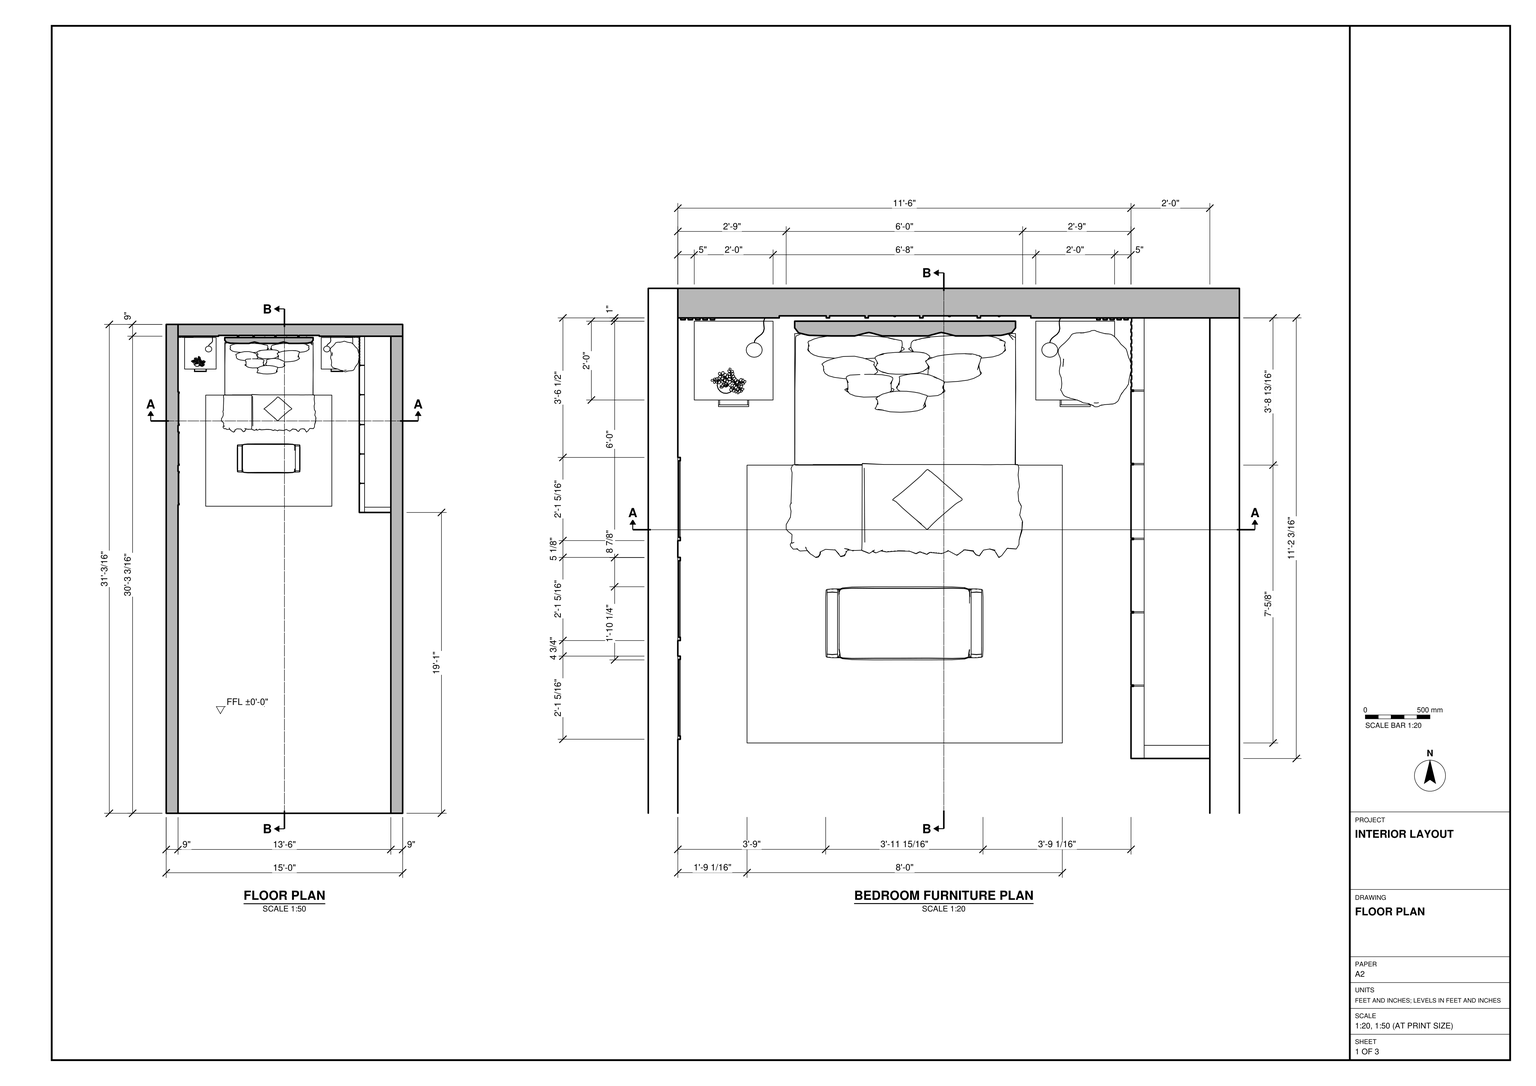
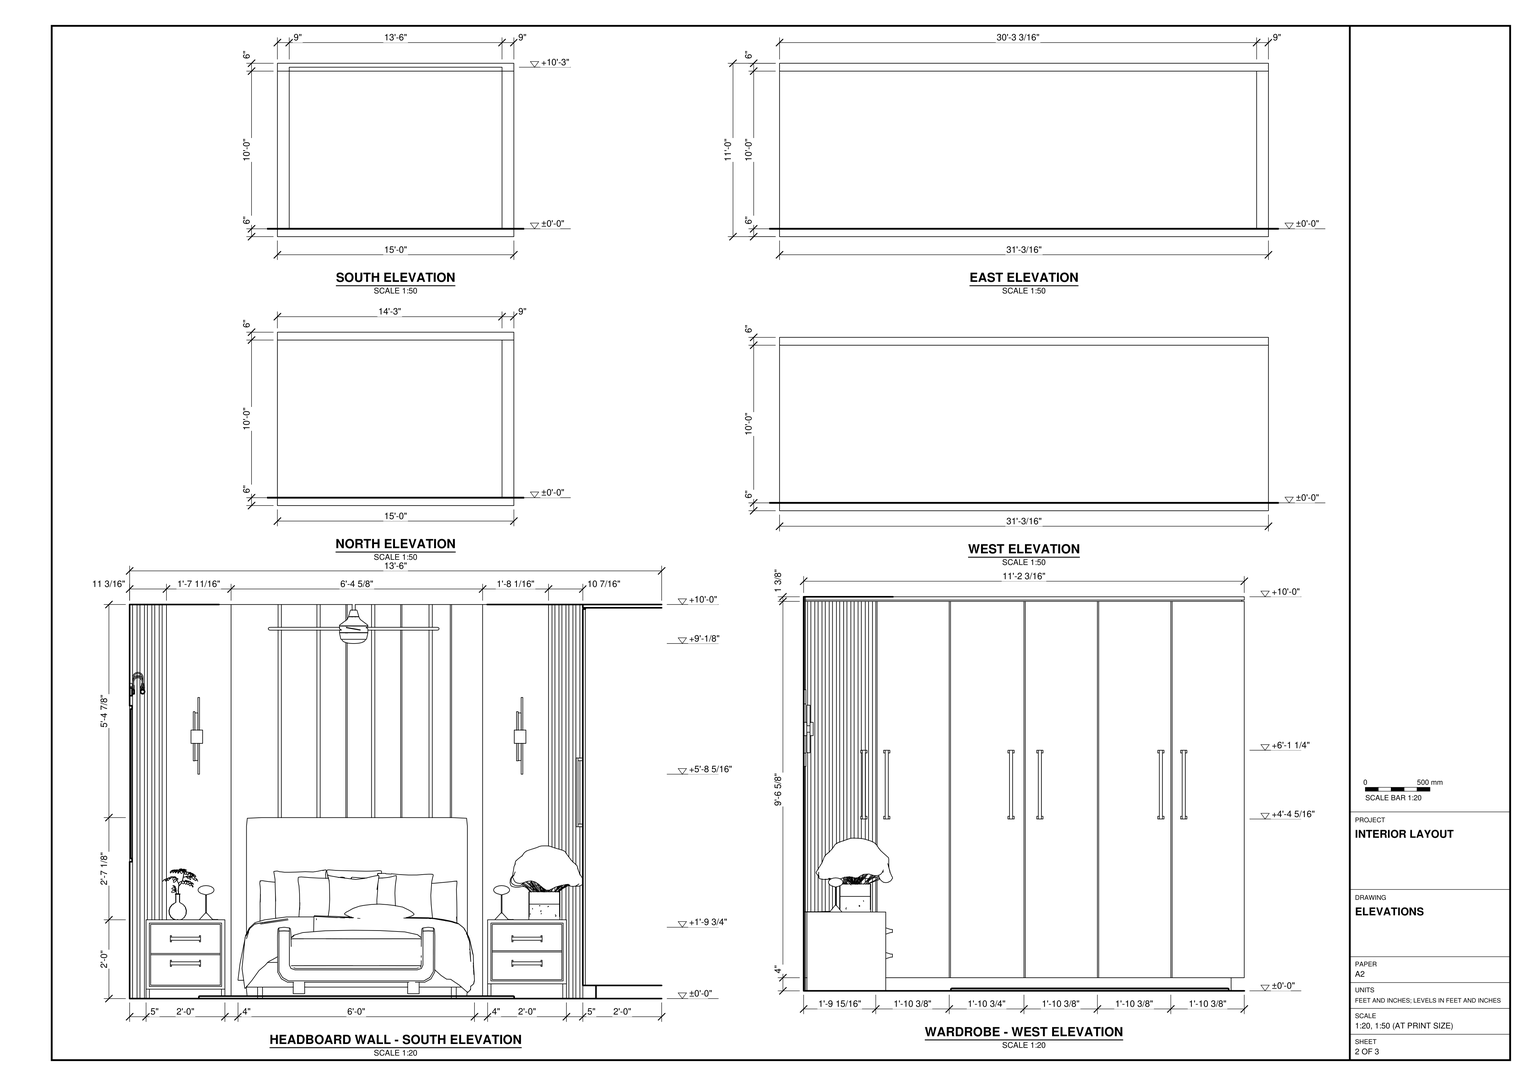
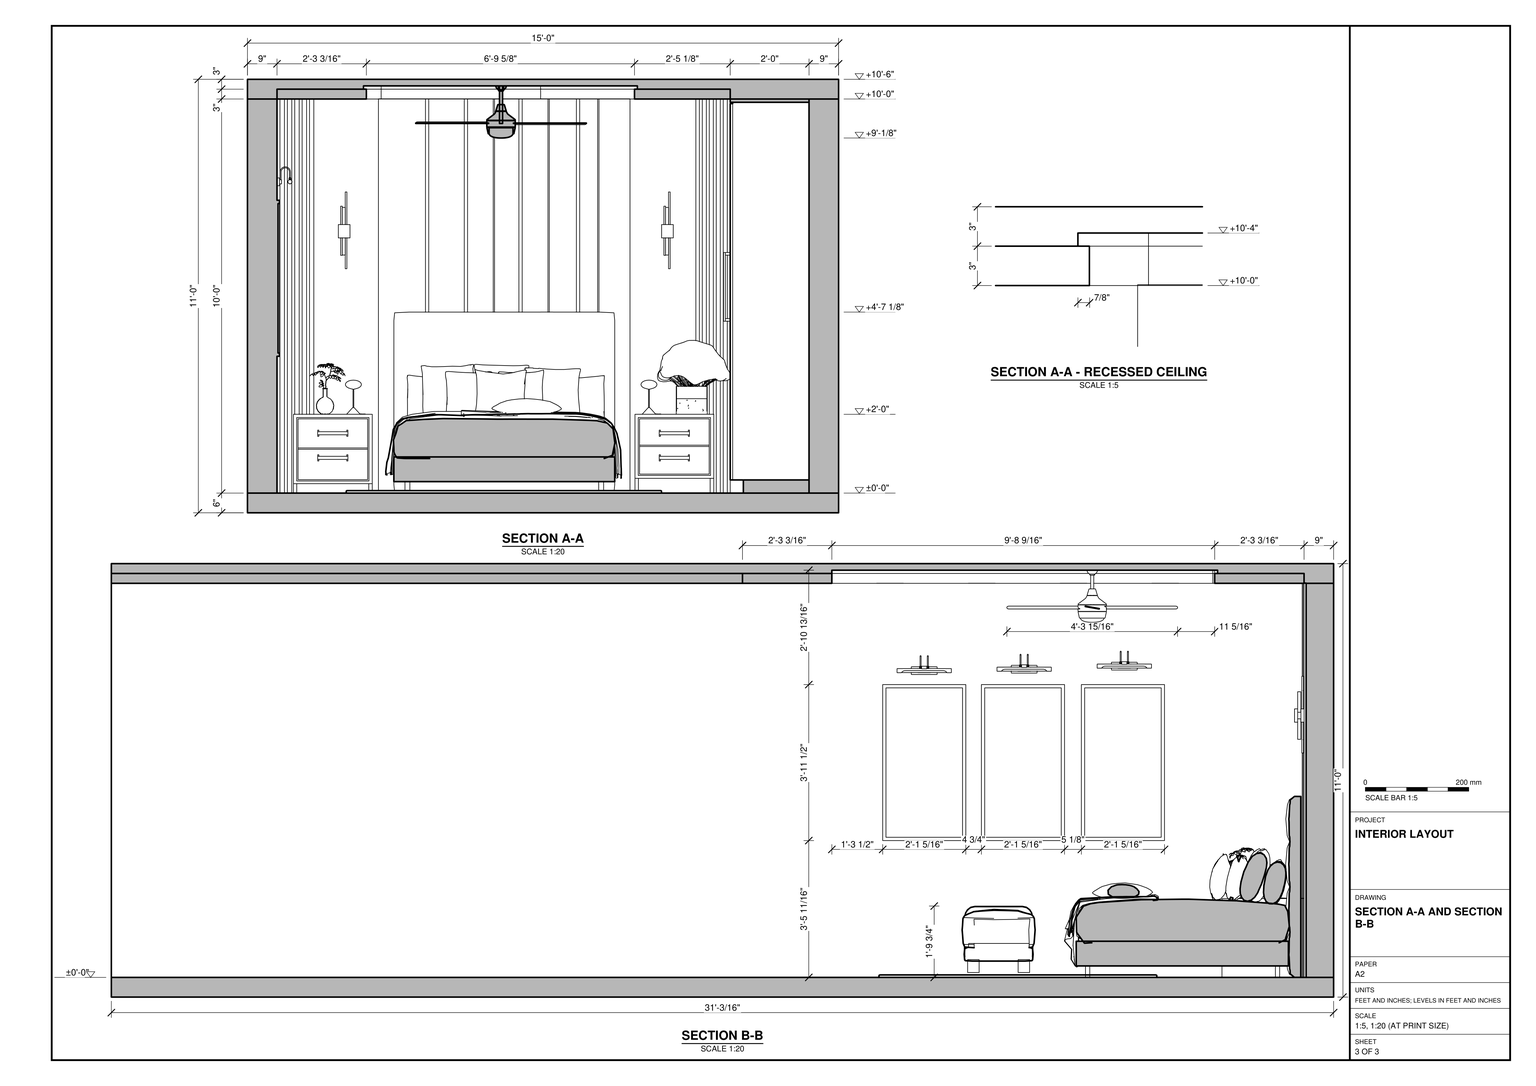
Work in feet and inches. Use task_files/diagram_01.pdf to build the bedroom in SketchUp. Set the finished floor at ±0'-0" and make the shell 15'-0" wide, 31'-3/16" long and 11'-0" high overall. Build the floor slab, the two long side walls, the headboard wall and the upper slab. Use the wall and slab thicknesses shown in section. Leave the end opposite the headboard open as drawn.

Use the enlarged furniture plan to place the bed between the bedside drawer units, with the fitted wardrobe running along the adjacent side wall. Centre the bench across the foot of the bed and place the rug beneath the bench and the foot of the bed. Keep the remaining length of the room clear. Follow the elevations for the headboard wall panelling, the wardrobe fronts, handles and recessed base. Use the sections to locate the stepped ceiling recess, ceiling fan, wall lights and framed panels.

Keep shell elements and individual furniture or joinery pieces in separate groups or components, and use components for repeated parts. Decor and loose items, including the rug, lamps and bedside objects, may be any suitable library components. Save one SketchUp model as output_files/bedroom_with_a_fitted_wardrobe_and_recessed_ceiling.skp.

# SketchUp Ruby script. Lengths in inches.
U = 1.inch
M = Sketchup.active_model
def pt(a) = Geom::Point3d.new(a.map { |v| v * U })
def face(e, loops, mat)
  f = e.add_face(loops[0].map { |a| pt(a) })
  loops[1..].each { |l| e.add_face(l.map { |a| pt(a) }).erase! }
  f.material = f.back_material = mat if mat
  f
end
# faces: each face lists its corners as indices into pts; further lists are holes
def faces(e, pts, list, mat = nil) = list.each { |f| face(e, (f[0].is_a?(Array) ? f : [f]).map { |l| l.map { |i| pts[i] } }, mat) }
# xy, xz, yz: faces in a plane at the given z, y or x. An outline is a flat list of corners, or four numbers for a rectangle; further outlines are holes
def ring(l) = l.size == 4 ? [[l[0], l[1]], [l[2], l[1]], [l[2], l[3]], [l[0], l[3]]] : l.each_slice(2).to_a
def flat(e, list, mat, &to3) = list.each { |f| face(e, (f[0].is_a?(Array) ? f : [f]).map { |l| ring(l).map { |u, v| to3.(u, v) } }, mat) }
def xy(e, z, list, mat = nil) = flat(e, list, mat) { |x, y| [x, y, z] }
def xz(e, y, list, mat = nil) = flat(e, list, mat) { |x, z| [x, y, z] }
def yz(e, x, list, mat = nil) = flat(e, list, mat) { |y, z| [x, y, z] }
def lines(e, pts, list) = list.each { |a, b| e.add_line(pt(pts[a]), pt(pts[b])) }
# prism: a flat outline (further loops are holes) pulled along v
def prism(e, loops, v, mat = nil)
  f = face(e, loops, mat); d = Geom::Vector3d.new(v.map { |x| x * U })
  f.pushpull(f.normal.samedirection?(d) ? d.length : -d.length)
end
def box(e, o, s, mat = nil) = prism(e, [[o, [o[0] + s[0], o[1], o[2]], [o[0] + s[0], o[1] + s[1], o[2]], [o[0], o[1] + s[1], o[2]]]], [0, 0, s[2]], mat)
def at(x, y, z, deg = 0) = Geom::Transformation.translation(pt([x, y, z])) * Geom::Transformation.rotation(ORIGIN, Z_AXIS, deg.degrees)
def axes(o, x, y, z) = Geom::Transformation.new([*x, 0, *y, 0, *z, 0, *pt(o).to_a, 1])
def part(name) = M.definitions.add(name)
# library, detail: a bought-in or finely detailed component or shape, given as its bounding box
def library(name, o, s) = part(name).tap { |d| box(d.entities, o, s) }
def detail(e, o, s) = box(e.add_group.entities, o, s)
def put(e, d, t, mat = nil) = e.add_instance(d, t).tap { |i| i.material = mat if mat }
def group(e, t, mat = nil) = e.add_group.tap { |g| g.transformation = t; g.material = mat if mat }.entities
root = M.entities
M.materials.add("Ashlee 5_ x 8_").color = [182, 173, 150]
M.materials.add("Emissive").color = [213, 214, 175]
M.materials.add("Generic").color = [224, 223, 223]
M.materials.add("Gold 10k").color = [251, 232, 180]
M.materials.add("Marble Crema Marfil 150cm").color = [157, 152, 147]
M.materials.add("[Color M03]").color = [170, 170, 170]
M.materials.add("[Wood Board Cork]").color = [215, 201, 115]
M.materials.add("[Wood Cherry Original]").color = [150, 85, 41]
M.materials.add("[Wood Floor]").color = [155, 105, 61]
M.materials.add("[Wood Veneer 02]").color = [188, 127, 90]
c1 = library("Bed 003",[-38.05,-87.1,0],[75.86,87.1,55.12])
c2 = library("Eva Bench",[-23.95,-11.14,0],[47.9,22.28,20.23])
c3 = library("Tlon Light 1950 Ceiling 152 010",[-38.39,-38.39,-3.78],[76.78,76.78,3.41])
c4 = library("Lamp Table 017",[-3.125,-3.125,0],[24.98,28.94,24.3125])
c5 = library("DenTuong JQ5640 (420mm)",[-8.27,0,0],[16.54,5.75,4.57])
c6 = library("marble wall light",[1.77,1.13,0],[2.91,3.55,23.375])
c7 = library("Ceiling_Fan_132cm",[44.98,-61.15,76.4375],[51.97,51.97,15.87])
c8 = part(" rug 5'x8'\#1")
xy(c8.entities,0,[[0,0,60,96]],"Ashlee 5_ x 8_")
xy(c8.entities,0.75,[[0.25,0.25,59.75,95.75]],"Ashlee 5_ x 8_")
xz(c8.entities,0,[[0,0,60,0.5]],"Ashlee 5_ x 8_")
xz(c8.entities,96,[[0,0,60,0.5]],"Ashlee 5_ x 8_")
yz(c8.entities,0,[[0,0,96,0.5]],"Ashlee 5_ x 8_")
yz(c8.entities,60,[[0,0,96,0.5]],"Ashlee 5_ x 8_")
p = [[59.99,0.01,0.56],[0.01,0.01,0.56],[0,0,0.5],[60,0,0.5],[0.01,95.99,0.56],[0,96,0.5],
  [59.99,95.99,0.56],[60,96,0.5],[0.03,0.03,0.625],[0.03,95.97,0.625],[59.97,0.03,0.625],[59.93,0.07,0.68],
  [0.07,0.07,0.68],[0.07,95.93,0.68],[59.93,95.93,0.68],[59.97,95.97,0.625],[0.125,0.125,0.72],[0.125,95.875,0.72],
  [59.81,0.19,0.74],[0.19,0.19,0.74],[59.875,0.125,0.72],[0.19,95.81,0.74],[59.81,95.81,0.74],[59.875,95.875,0.72],
  [0.25,0.25,0.75],[0.25,95.75,0.75],[59.75,0.25,0.75],[59.75,95.75,0.75]]
faces(c8.entities,p,[[0,1,2,3],[1,4,5,2],[6,0,3,7],[4,6,7,5],[8,9,4,1],[10,8,1,0],[11,12,8,10],[12,13,9,8],
  [14,11,10,15],[15,10,0,6],[13,14,15,9],[9,15,6,4],[16,17,13,12],[18,19,16,20],[20,16,12,11],[19,21,17,16],
  [22,18,20,23],[23,20,11,14],[24,25,21,19],[26,24,19,18],[27,26,18,22],[21,22,23,17],[25,27,22,21],[17,23,14,13]],"Ashlee 5_ x 8_")
c9 = library("Vase Roses 63-11",[-11.16,-11.66,0.01],[22.4,23.28,22.51])
c10 = library("Vase 111-18",[-4.54,-2.8,0.01],[10.64,7.87,15.5])
c11 = part("POI-E1497-320-1917\#1")
xy(c11.entities,0,[[0,0,0.29,0.83],[7.21,0,7.5,0.83]])
xy(c11.entities,0.64,[[0.29,0.21,7.21,0.62]])
xy(c11.entities,0.875,[[0,0.21,7.5,0.62]])
xz(c11.entities,0.21,[[0,0.64,7.5,0.875]])
xz(c11.entities,0.62,[[0,0.64,7.5,0.875]])
yz(c11.entities,0,[[0,0,0.21,0.64,0.21,0.875,0.62,0.875,0.62,0.64,0.83,0]])
yz(c11.entities,0.29,[[0,0,0.83,0,0.62,0.64,0.21,0.64]])
yz(c11.entities,7.21,[[0,0,0.21,0.64,0.62,0.64,0.83,0]])
yz(c11.entities,7.5,[[0,0,0.83,0,0.62,0.64,0.62,0.875,0.21,0.875,0.21,0.64]])
p = [[0,0.21,0.64],[0,0,0],[0.29,0,0],[0.29,0.21,0.64],[7.21,0.21,0.64],[7.21,0,0],
  [7.5,0,0],[7.5,0.21,0.64],[0,0.83,0],[0,0.62,0.64],[0.29,0.62,0.64],[0.29,0.83,0],
  [7.5,0.83,0],[7.5,0.62,0.64],[7.21,0.62,0.64],[7.21,0.83,0]]
faces(c11.entities,p,[[0,1,2,3],[4,5,6,7],[8,9,10,11],[12,13,14,15]])
xy(root,-6,[[0,0,180,372.1875]])
xy(root,0,[[0,0,9,372.1875],[171,0,180,363.1875],[151,233.02,171,233.02,171,363.1875,180,363.1875,180,372.1875,9,372.1875,9,363.1875,9.9,363.1875,9.9,362.625,11.25,362.625,11.25,363.1875,12.15,363.1875,12.15,362.625,13.5,362.625,13.5,363.1875,14.4,363.1875,14.4,362.625,15.75,362.625,15.75,363.1875,16.65,363.1875,16.65,362.625,18,362.625,18,363.1875,18.9,363.1875,18.9,362.625,20.21,362.625,20.21,363.1875,39.88,363.1875,39.88,363.8125,54.2,363.8125,54.2,363.1875,55.2,363.1875,55.2,363.8125,66.02,363.8125,66.02,363.1875,67.02,363.1875,67.02,363.8125,74.84,363.8125,74.84,363.625,75.24,363.625,75.24,363.8125,82.66,363.8125,82.66,363.1875,83.66,363.1875,83.66,363.8125,91.51,363.8125,91.51,363.625,91.91,363.625,91.91,363.8125,100.16,363.8125,100.16,363.1875,101.16,363.1875,101.16,363.8125,106.63,363.8125,106.63,363.625,107.03,363.625,107.03,363.8125,116.48,363.8125,116.48,363.1875,136.54,363.1875,136.54,362.625,137.6,362.625,137.6,363.1875,138.5,363.1875,138.5,362.625,139.73,362.625,139.73,363.1875,140.625,363.1875,140.625,362.625,141.85,362.625,141.85,363.1875,142.75,363.1875,142.75,362.625,143.98,362.625,143.98,363.1875,144.875,363.1875,144.875,362.625,146.1,362.625,146.1,363.1875,151,363.1875],[151,233.02,171,363.1875],[14,338.1875,14,362.1875,38,362.1875,38,338.1875,36.94,338.1875,36.94,360.1875,15.02,360.1875,15.02,338.1875],
  [118,338.1875,118,362.1875,142,362.1875,142,338.1875,140.89,338.1875,140.89,360.1875,119.03,360.1875,119.03,338.1875],[9.9,362.625,11.25,363.1875],[12.15,362.625,13.5,363.1875],[14.4,362.625,15.75,363.1875],[16.65,362.625,18,363.1875],
  [18.9,362.625,20.21,363.1875],[136.54,362.625,137.6,363.1875],[138.5,362.625,139.73,363.1875],[140.625,362.625,141.85,363.1875],[142.75,362.625,143.98,363.1875],
  [144.875,362.625,146.1,363.1875],[9,363.1875,9,372.1875,180,372.1875,180,363.1875,116.48,363.1875,116.48,363.8125,101.16,363.8125,101.16,363.1875,100.16,363.1875,100.16,363.8125,83.66,363.8125,83.66,363.1875,82.66,363.1875,82.66,363.8125,67.02,363.8125,67.02,363.1875,66.02,363.1875,66.02,363.8125,55.2,363.8125,55.2,363.1875,54.2,363.1875,54.2,363.8125,39.88,363.8125,39.88,363.1875],[74.84,363.625,75.24,363.8125],[91.51,363.625,91.91,363.8125],[106.63,363.625,107.03,363.8125]])
xy(root,0,[[[9,0,171,0,171,233.02,151,233.02,151,363.1875,146.1,363.1875,146.1,362.625,144.875,362.625,144.875,363.1875,143.98,363.1875,143.98,362.625,142.75,362.625,142.75,363.1875,141.85,363.1875,141.85,362.625,140.625,362.625,140.625,363.1875,139.73,363.1875,139.73,362.625,138.5,362.625,138.5,363.1875,137.6,363.1875,137.6,362.625,136.54,362.625,136.54,363.1875,116.48,363.1875,116.48,363.8125,107.03,363.8125,107.03,363.625,106.63,363.625,106.63,363.8125,101.16,363.8125,101.16,363.1875,100.16,363.1875,100.16,363.8125,91.91,363.8125,91.91,363.625,91.51,363.625,91.51,363.8125,83.66,363.8125,83.66,363.1875,82.66,363.1875,82.66,363.8125,75.24,363.8125,75.24,363.625,74.84,363.625,74.84,363.8125,67.02,363.8125,67.02,363.1875,66.02,363.1875,66.02,363.8125,55.2,363.8125,55.2,363.1875,54.2,363.1875,54.2,363.8125,39.88,363.8125,39.88,363.1875,20.21,363.1875,20.21,362.625,18.9,362.625,18.9,363.1875,18,363.1875,18,362.625,16.65,362.625,16.65,363.1875,15.75,363.1875,15.75,362.625,14.4,362.625,14.4,363.1875,13.5,363.1875,13.5,362.625,12.15,362.625,12.15,363.1875,11.25,363.1875,11.25,362.625,9.9,362.625,9.9,363.1875,9,363.1875],[118,338.1875,118,362.1875,142,362.1875,142,338.1875,140.89,338.1875,140.89,360.1875,119.03,360.1875,119.03,338.1875],[14,338.1875,14,362.1875,38,362.1875,38,338.1875,36.94,338.1875,36.94,360.1875,15.02,360.1875,15.02,338.1875]]],"Marble Crema Marfil 150cm")
xy(root,2.87,[[15.02,338.1875,36.94,360.1875]])
xy(root,3.6875,[[15,338.1875,37,338.9375]],"Gold 10k")
xy(root,4,[[151,233.02,171,363.1875],[147.75,250.98,151,251.38],[147,251.38,151,273.34],[147.75,273.34,151,273.74],[147,273.74,151,295.7],
  [147.75,295.7,151,296.1],[147,296.1,151,318.46],[147.75,318.46,151,318.86],[147,318.86,151,340.83],[147.75,340.83,151,341.23],
  [147,341.23,147,342.23,147.1875,342.23,147.1875,343.42,147,343.42,147,344.42,147.1875,344.42,147.1875,345.62,147,345.62,147,346.62,147.1875,346.62,147.1875,347.81,147,347.81,147,348.81,147.1875,348.81,147.1875,350.01,147,350.01,147,351.01,147.1875,351.01,147.1875,352.21,147,352.21,147,353.21,147.1875,353.21,147.1875,354.4,147,354.4,147,355.4,147.1875,355.4,147.1875,356.6,147,356.6,147,357.6,147.1875,357.6,147.1875,358.8,147,358.8,147,359.8,147.1875,359.8,147.1875,360.99,147,360.99,147,361.99,147.1875,361.99,147.1875,363.1875,151,363.1875,151,341.23]])
xy(root,4,[[147,229.02,151,250.98],[151,229.02,171,233.02]],"Gold 10k")
xy(root,4.09,[[15.4,338.1875,36.6,338.9375]])
xy(root,4.49,[[119.03,338.1875,140.89,360.1875]])
xy(root,5.375,[[119,338.1875,141,338.9375]],"Gold 10k")
xy(root,5.78,[[119.4,338.1875,140.6,338.9375]],"Gold 10k")
xy(root,13.34,[[15.4,338.1875,36.6,338.9375]],"Gold 10k")
xy(root,13.74,[[15.4,338.1875,36.6,338.9375]],"Gold 10k")
xy(root,14.1875,[[119.4,338.1875,140.6,338.9375]],"Gold 10k")
xy(root,14.59,[[119.4,338.1875,140.6,338.9375]],"Gold 10k")
xy(root,22.6,[[15.4,338.1875,36.6,338.9375],[119.4,338.1875,140.6,338.9375]],"Gold 10k")
xy(root,23,[[15,338.1875,37,338.9375],[119,338.1875,141,338.9375]],"Gold 10k")
xy(root,24,[[14,338.1875,38,362.1875],[118,338.1875,142,362.1875]],"Generic")
xy(root,41.66,[[9,234.875,9.75,260.1875],[9,264.9375,9.75,290.25],[9,295.375,9.75,320.6875]],"[Wood Board Cork]")
xy(root,42.66,[[9.3125,235.875,9.75,259.1875],[9.3125,265.9375,9.75,289.25],[9.3125,296.375,9.75,319.6875]],"[Wood Board Cork]")
xy(root,88.16,[[9.3125,235.875,9.75,259.1875],[9.3125,265.9375,9.75,289.25],[9.3125,296.375,9.75,319.6875]],"[Wood Board Cork]")
xy(root,89.16,[[9,234.875,9.75,260.1875],[9,264.9375,9.75,290.25],[9,295.375,9.75,320.6875]],"[Wood Board Cork]")
xy(root,118.6,[[147,273.74,147.75,295.7],[147,296.1,147.75,318.46]])
xy(root,118.6,[[147,229.02,147.75,250.98],[147.75,229.02,171,229.77],[147,251.38,147.75,273.34],[147,318.86,147.75,340.83],[147,341.23,147.75,341.23,147.75,363.1875,147.1875,363.1875,147.1875,361.99,147,361.99,147,360.99,147.1875,360.99,147.1875,359.8,147,359.8,147,358.8,147.1875,358.8,147.1875,357.6,147,357.6,147,356.6,147.1875,356.6,147.1875,355.4,147,355.4,147,354.4,147.1875,354.4,147.1875,353.21,147,353.21,147,352.21,147.1875,352.21,147.1875,351.01,147,351.01,147,350.01,147.1875,350.01,147.1875,348.81,147,348.81,147,347.81,147.1875,347.81,147.1875,346.62,147,346.62,147,345.62,147.1875,345.62,147.1875,344.42,147,344.42,147,343.42,147.1875,343.42,147.1875,342.23,147,342.23]],"Gold 10k")
xy(root,119,[[147.75,229.77,171,363.1875]])
xy(root,119,[[147,229.02,147.75,363.1875],[147.75,229.02,171,229.77]],"Gold 10k")
xy(root,120,[[0,0,9,372.1875],[9,0,171,192.1875],[171,0,180,363.1875],[147,229.02,171,363.1875],[9.9,362.625,11.25,363.1875],
  [12.15,362.625,13.5,363.1875],[14.4,362.625,15.75,363.1875],[16.65,362.625,18,363.1875],[18.9,362.625,20.21,363.1875],[136.54,362.625,137.6,363.1875],
  [138.5,362.625,139.73,363.1875],[140.625,362.625,141.85,363.1875],[142.75,362.625,143.98,363.1875],[144.875,362.625,146.1,363.1875],[9,363.1875,9,372.1875,180,372.1875,180,363.1875,116.48,363.1875,116.48,363.8125,39.88,363.8125,39.88,363.1875],
  [54.2,363.1875,55.2,363.8125],[66.02,363.1875,67.02,363.8125],[82.66,363.1875,83.66,363.8125],[100.16,363.1875,101.16,363.8125],[74.84,363.625,75.24,363.8125],
  [91.51,363.625,91.91,363.8125],[106.63,363.625,107.03,363.8125]])
xy(root,120,[[[9,192.1875,9,363.1875,9.9,363.1875,9.9,362.625,11.25,362.625,11.25,363.1875,12.15,363.1875,12.15,362.625,13.5,362.625,13.5,363.1875,14.4,363.1875,14.4,362.625,15.75,362.625,15.75,363.1875,16.65,363.1875,16.65,362.625,18,362.625,18,363.1875,18.9,363.1875,18.9,362.625,20.21,362.625,20.21,363.1875,136.54,363.1875,136.54,362.625,137.6,362.625,137.6,363.1875,138.5,363.1875,138.5,362.625,139.73,362.625,139.73,363.1875,140.625,363.1875,140.625,362.625,141.85,362.625,141.85,363.1875,142.75,363.1875,142.75,362.625,143.98,362.625,143.98,363.1875,144.875,363.1875,144.875,362.625,146.1,362.625,146.1,363.1875,147,363.1875,147,229.02,171,229.02,171,192.1875],[36.21,219.4,117.85,219.4,117.85,335.98,89.27,335.98,40.71,335.41,36.21,335.41]]],"[Color M03]")
xy(root,120.0625,[[39.88,363.1875,116.48,363.8125]],"Emissive")
xy(root,123,[[9,0,171,192.1875],[[9,192.1875,171,192.1875,171,229.02,147,229.02,147,363.1875,146.1,363.1875,146.1,362.625,144.875,362.625,144.875,363.1875,143.98,363.1875,143.98,362.625,142.75,362.625,142.75,363.1875,141.85,363.1875,141.85,362.625,140.625,362.625,140.625,363.1875,139.73,363.1875,139.73,362.625,138.5,362.625,138.5,363.1875,137.6,363.1875,137.6,362.625,136.54,362.625,136.54,363.1875,20.21,363.1875,20.21,362.625,18.9,362.625,18.9,363.1875,18,363.1875,18,362.625,16.65,362.625,16.65,363.1875,15.75,363.1875,15.75,362.625,14.4,362.625,14.4,363.1875,13.5,363.1875,13.5,362.625,12.15,362.625,12.15,363.1875,11.25,363.1875,11.25,362.625,9.9,362.625,9.9,363.1875,9,363.1875],[35.34,219.4,35.34,336.29,40.71,336.29,40.71,335.41,89.27,335.98,89.27,336.85,118.73,336.85,118.73,219.4]]])
xy(root,123,[[35.34,219.4,36.21,336.29],[117.85,219.4,118.73,336.85],[36.21,335.41,40.71,336.29],[89.27,335.98,117.85,336.85]],"Emissive")
xy(root,124,[[35.34,219.4,35.34,336.29,40.71,336.29,40.71,335.41,89.27,335.98,89.27,336.85,118.73,336.85,118.73,219.4]],"[Color M03]")
xy(root,126,[[0,0,180,372.1875]])
xz(root,0,[[0,-6,180,0],[0,0,9,120],[9,0,171,120],[171,0,180,120],[0,120,9,120,9,123,171,123,171,120,180,120,180,126,0,126],
  [9,120,171,123]])
xz(root,192.1875,[[9,120,171,123]])
xz(root,219.4,[[36.21,120,117.85,123]])
xz(root,219.4,[[35.34,123,118.73,124]],"Emissive")
xz(root,229.02,[[147,120,171,123]])
xz(root,229.02,[[147,4,171,118.6]],"Generic")
xz(root,229.02,[[147,119,171,120]],"[Wood Floor]")
xz(root,229.77,[[147.75,118.6,171,119]],"Gold 10k")
xz(root,233.02,[[151,0,171,4]],"Gold 10k")
xz(root,234.875,[[9,41.66,9.75,89.16]],"[Wood Board Cork]")
xz(root,235.875,[[9.3125,42.66,9.75,88.16]],"[Wood Board Cork]")
xz(root,250.98,[[147,4,147.75,118.6]],"Gold 10k")
xz(root,251.38,[[147,4,147.75,118.6]],"Gold 10k")
xz(root,259.1875,[[9.3125,42.66,9.75,88.16]],"[Wood Board Cork]")
xz(root,260.1875,[[9,41.66,9.75,89.16]],"[Wood Board Cork]")
xz(root,264.9375,[[9,41.66,9.75,89.16]],"[Wood Board Cork]")
xz(root,265.9375,[[9.3125,42.66,9.75,88.16]],"[Wood Board Cork]")
xz(root,273.34,[[147,4,147.75,118.6]],"Gold 10k")
xz(root,273.74,[[147,4,147.75,118.6]],"Gold 10k")
xz(root,289.25,[[9.3125,42.66,9.75,88.16]],"[Wood Board Cork]")
xz(root,290.25,[[9,41.66,9.75,89.16]],"[Wood Board Cork]")
xz(root,295.375,[[9,41.66,9.75,89.16]],"[Wood Board Cork]")
xz(root,295.7,[[147,4,147.75,118.6]],"Gold 10k")
xz(root,296.1,[[147,4,147.75,118.6]],"Gold 10k")
xz(root,296.375,[[9.3125,42.66,9.75,88.16]],"[Wood Board Cork]")
xz(root,318.46,[[147,4,147.75,118.6]],"Gold 10k")
xz(root,318.86,[[147,4,147.75,118.6]],"Gold 10k")
xz(root,319.6875,[[9.3125,42.66,9.75,88.16]],"[Wood Board Cork]")
xz(root,320.6875,[[9,41.66,9.75,89.16]],"[Wood Board Cork]")
xz(root,335.41,[[36.21,120,40.71,123]],"[Color M03]")
xz(root,335.98,[[89.27,120,117.85,123]],"[Color M03]")
xz(root,336.29,[[35.34,123,40.71,124]],"Emissive")
xz(root,336.85,[[89.27,123,118.73,124]],"Emissive")
xz(root,338.1875,[[[14,2.87,38,24],[15,3.6875,37,23]],[15.4,4.09,36.6,13.34],[[118,4.49,142,24],[119,5.375,141,23]],[119.4,5.78,140.6,14.1875],[15.4,13.74,36.6,22.6],
  [119.4,14.59,140.6,22.6]],"Generic")
xz(root,338.1875,[[14,0,15.02,2.87],[36.94,0,38,2.87],[118,0,119.03,4.49],[140.89,0,142,4.49]],"Gold 10k")
xz(root,338.9375,[[[15,3.6875,37,23],[15.4,4.09,36.6,22.6]],[[119,5.375,141,23],[119.4,5.78,140.6,22.6]],[15.4,13.34,36.6,13.74],[119.4,14.1875,140.6,14.59]],"Gold 10k")
xz(root,340.83,[[147,4,147.75,118.6]],"Gold 10k")
xz(root,341.23,[[147,4,147.75,118.6]],"Gold 10k")
xz(root,342.23,[[147,4,147.1875,118.6]])
xz(root,343.42,[[147,4,147.1875,118.6]],"Gold 10k")
xz(root,344.42,[[147,4,147.1875,118.6]])
xz(root,345.62,[[147,4,147.1875,118.6]],"Gold 10k")
xz(root,346.62,[[147,4,147.1875,118.6]])
xz(root,347.81,[[147,4,147.1875,118.6]],"Gold 10k")
xz(root,348.81,[[147,4,147.1875,118.6]])
xz(root,350.01,[[147,4,147.1875,118.6]],"Gold 10k")
xz(root,351.01,[[147,4,147.1875,118.6]])
xz(root,352.21,[[147,4,147.1875,118.6]],"Gold 10k")
xz(root,353.21,[[147,4,147.1875,118.6]])
xz(root,354.4,[[147,4,147.1875,118.6]],"Gold 10k")
xz(root,355.4,[[147,4,147.1875,118.6]],"Gold 10k")
xz(root,356.6,[[147,4,147.1875,118.6]],"Gold 10k")
xz(root,357.6,[[147,4,147.1875,118.6]],"Gold 10k")
xz(root,358.8,[[147,4,147.1875,118.6]],"Gold 10k")
xz(root,359.8,[[147,4,147.1875,118.6]],"Gold 10k")
xz(root,360.1875,[[15.02,0,36.94,2.87],[119.03,0,140.89,4.49]])
xz(root,360.99,[[147,4,147.1875,118.6]],"Gold 10k")
xz(root,361.99,[[147,4,147.1875,118.6]],"Gold 10k")
xz(root,362.1875,[[14,0,38,24],[118,0,142,24]])
xz(root,362.625,[[9.9,120,11.25,123],[12.15,120,13.5,123],[14.4,120,15.75,123],[16.65,120,18,123],[18.9,120,20.21,123],
  [136.54,120,137.6,123],[138.5,120,139.73,123],[140.625,120,141.85,123],[142.75,120,143.98,123],[144.875,120,146.1,123]])
xz(root,362.625,[[9.9,0,11.25,120],[12.15,0,13.5,120],[14.4,0,15.75,120],[16.65,0,18,120],[18.9,0,20.21,120],
  [136.54,0,137.6,120],[138.5,0,139.73,120],[140.625,0,141.85,120],[142.75,0,143.98,120],[144.875,0,146.1,120]],"[Wood Floor]")
xz(root,363.1875,[[9.9,0,11.25,120],[12.15,0,13.5,120],[14.4,0,15.75,120],[16.65,0,18,120],[18.9,0,20.21,120],
  [136.54,0,137.6,120],[138.5,0,139.73,120],[140.625,0,141.85,120],[142.75,0,143.98,120],[144.875,0,146.1,120],
  [151,0,171,4],[171,0,180,120],[147.1875,4,171,4,171,119,147.75,119,147.75,118.6,147.1875,118.6],[147,119,171,120],[9,120,9.9,123],
  [11.25,120,12.15,123],[13.5,120,14.4,123],[15.75,120,16.65,123],[18,120,18.9,123],[20.21,120,39.88,123],
  [54.2,120,55.2,120.0625],[55.2,120,66.02,120.0625],[66.02,120,67.02,120.0625],[67.02,120,82.66,120.0625],[82.66,120,83.66,120.0625],
  [83.66,120,100.16,120.0625],[100.16,120,101.16,120.0625],[101.16,120,116.48,120.0625],[116.48,120,136.54,123],[137.6,120,138.5,123],
  [139.73,120,140.625,123],[141.85,120,142.75,123],[143.98,120,144.875,123],[146.1,120,147,123],[39.88,120.0625,54.2,123],
  [54.2,120.0625,55.2,123],[55.2,120.0625,66.02,123],[66.02,120.0625,67.02,123],[67.02,120.0625,82.66,123],[82.66,120.0625,83.66,123],
  [83.66,120.0625,100.16,123],[100.16,120.0625,101.16,123],[101.16,120.0625,116.48,123]])
xz(root,363.1875,[[39.88,120,54.2,120.0625]],"Emissive")
xz(root,363.1875,[[54.2,0,55.2,120],[66.02,0,67.02,120],[82.66,0,83.66,120],[100.16,0,101.16,120]],"Gold 10k")
xz(root,363.1875,[[20.21,0,39.88,120],[116.48,0,136.54,120]],"[Wood Cherry Original]")
xz(root,363.1875,[[9,0,9.9,120],[11.25,0,12.15,120],[13.5,0,14.4,120],[15.75,0,16.65,120],[18,0,18.9,120],
  [137.6,0,138.5,120],[139.73,0,140.625,120],[141.85,0,142.75,120],[143.98,0,144.875,120],[146.1,0,147,120],
  [147,0,151,0,151,4,147.1875,4,147.1875,118.6,147.75,118.6,147.75,119,147,119]],"[Wood Floor]")
xz(root,363.625,[[74.84,0,75.24,120],[91.51,0,91.91,120],[106.63,0,107.03,120]],"[Color M03]")
xz(root,363.8125,[[74.84,0,75.24,120],[91.51,0,91.91,120],[106.63,0,107.03,120]])
xz(root,363.8125,[[39.88,120,116.48,120.0625]],"Emissive")
xz(root,363.8125,[[39.88,0,54.2,120],[55.2,0,66.02,120],[67.02,0,74.84,120],[75.24,0,82.66,120],[83.66,0,91.51,120],
  [91.91,0,100.16,120],[101.16,0,106.63,120],[107.03,0,116.48,120]],"[Color M03]")
xz(root,372.1875,[[0,-6,180,0],[0,0,9,120],[9,0,180,120],[0,120,180,126]])
yz(root,0,[[0,-6,372.1875,0],[0,0,372.1875,120],[0,120,372.1875,126]])
yz(root,9,[[363.1875,0,372.1875,120],[0,120,192.1875,123],[192.1875,120,363.1875,123]])
yz(root,9,[[[0,0,363.1875,120],[295.375,41.66,320.6875,89.16],[264.9375,41.66,290.25,89.16],[234.875,41.66,260.1875,89.16]]],"[Color M03]")
yz(root,9.3125,[[235.875,42.66,259.1875,88.16],[265.9375,42.66,289.25,88.16],[296.375,42.66,319.6875,88.16]],"[Wood Veneer 02]")
yz(root,9.75,[[[234.875,41.66,260.1875,89.16],[235.875,42.66,259.1875,88.16]],[[264.9375,41.66,290.25,89.16],[265.9375,42.66,289.25,88.16]],[[295.375,41.66,320.6875,89.16],[296.375,42.66,319.6875,88.16]]],"[Wood Board Cork]")
yz(root,9.9,[[362.625,120,363.1875,123]])
yz(root,9.9,[[362.91,0,363.1875,120]],"Emissive")
yz(root,9.9,[[362.625,0,362.91,120]],"[Wood Floor]")
yz(root,11.25,[[362.625,120,363.1875,123]])
yz(root,11.25,[[362.625,0,363.1875,120]],"[Wood Floor]")
yz(root,12.15,[[362.625,120,363.1875,123]])
yz(root,12.15,[[362.625,0,363.1875,120]],"[Wood Floor]")
yz(root,13.5,[[362.625,120,363.1875,123]])
yz(root,13.5,[[362.625,0,363.1875,120]],"[Wood Floor]")
yz(root,14,[[338.1875,0,362.1875,24]],"Generic")
yz(root,14.4,[[362.625,120,363.1875,123]])
yz(root,14.4,[[362.625,0,363.1875,120]],"[Wood Floor]")
yz(root,15,[[338.1875,3.6875,338.9375,23]],"Gold 10k")
yz(root,15.02,[[338.1875,0,360.1875,2.87]],"Gold 10k")
yz(root,15.4,[[338.1875,4.09,338.9375,13.34],[338.1875,13.74,338.9375,22.6]])
yz(root,15.75,[[362.625,120,363.1875,123]])
yz(root,15.75,[[362.625,0,363.1875,120]],"[Wood Floor]")
yz(root,16.65,[[362.625,120,363.1875,123]])
yz(root,16.65,[[362.625,0,363.1875,120]],"[Wood Floor]")
yz(root,18,[[362.625,120,363.1875,123]])
yz(root,18,[[362.625,0,363.1875,120]],"[Wood Floor]")
yz(root,18.9,[[362.625,120,363.1875,123]])
yz(root,18.9,[[362.625,0,363.1875,120]],"[Wood Floor]")
yz(root,20.21,[[362.625,120,363.1875,123]])
yz(root,20.21,[[362.91,0,363.1875,120]],"Emissive")
yz(root,20.21,[[362.625,0,362.91,120]],"[Wood Floor]")
yz(root,35.34,[[219.4,123,336.29,124]],"Emissive")
yz(root,36.21,[[219.4,120,335.41,123]],"[Color M03]")
yz(root,36.6,[[338.1875,4.09,338.9375,13.34],[338.1875,13.74,338.9375,22.6]],"Gold 10k")
yz(root,36.94,[[338.1875,0,360.1875,2.87]],"Gold 10k")
yz(root,37,[[338.1875,3.6875,338.9375,23]],"Gold 10k")
yz(root,38,[[338.1875,0,362.1875,24]],"Generic")
yz(root,39.88,[[363.1875,0,363.8125,120],[363.1875,120,363.8125,120.0625]],"Emissive")
yz(root,40.71,[[335.41,123,336.29,124]],"Emissive")
yz(root,54.2,[[363.1875,0,363.8125,120]],"Gold 10k")
yz(root,55.2,[[363.1875,0,363.8125,120]],"Gold 10k")
yz(root,66.02,[[363.1875,0,363.8125,120]],"Gold 10k")
yz(root,67.02,[[363.1875,0,363.8125,120]],"Gold 10k")
yz(root,74.84,[[363.625,0,363.8125,120]],"[Color M03]")
yz(root,75.24,[[363.625,0,363.8125,120]],"[Color M03]")
yz(root,82.66,[[363.1875,0,363.8125,120]],"Gold 10k")
yz(root,83.66,[[363.1875,0,363.8125,120]],"Gold 10k")
yz(root,89.27,[[335.98,123,336.85,124]],"Emissive")
yz(root,91.51,[[363.625,0,363.8125,120]])
yz(root,91.91,[[363.625,0,363.8125,120]],"[Color M03]")
yz(root,100.16,[[363.1875,0,363.8125,120]],"Gold 10k")
yz(root,101.16,[[363.1875,0,363.8125,120]],"Gold 10k")
yz(root,106.63,[[363.625,0,363.8125,120]],"[Color M03]")
yz(root,107.03,[[363.625,0,363.8125,120]],"[Color M03]")
yz(root,116.48,[[363.1875,0,363.8125,120],[363.1875,120,363.8125,120.0625]],"Emissive")
yz(root,117.85,[[219.4,120,335.98,123]],"[Color M03]")
yz(root,118,[[338.1875,0,362.1875,24]],"Generic")
yz(root,118.73,[[219.4,123,336.85,124]],"Emissive")
yz(root,119,[[338.1875,5.375,338.9375,23]],"Gold 10k")
yz(root,119.03,[[338.1875,0,360.1875,4.49]],"Gold 10k")
yz(root,119.4,[[338.1875,5.78,338.9375,14.1875],[338.1875,14.59,338.9375,22.6]],"Gold 10k")
yz(root,136.54,[[362.625,120,363.1875,123]])
yz(root,136.54,[[362.91,0,363.1875,120]],"Emissive")
yz(root,136.54,[[362.625,0,362.91,120]],"[Wood Floor]")
yz(root,137.6,[[362.625,120,363.1875,123]])
yz(root,137.6,[[362.625,0,363.1875,120]],"[Wood Floor]")
yz(root,138.5,[[362.625,119,363.1875,120],[362.625,120,363.1875,123]])
yz(root,138.5,[[362.625,0,363.1875,119]],"[Wood Floor]")
yz(root,139.73,[[362.625,120,363.1875,123]])
yz(root,139.73,[[362.625,0,363.1875,120]],"[Wood Floor]")
yz(root,140.6,[[338.1875,5.78,338.9375,14.1875],[338.1875,14.59,338.9375,22.6]])
yz(root,140.625,[[362.625,119,363.1875,120],[362.625,120,363.1875,123]])
yz(root,140.625,[[362.625,0,363.1875,119]],"[Wood Floor]")
yz(root,140.89,[[338.1875,0,360.1875,4.49]],"Gold 10k")
yz(root,141,[[338.1875,5.375,338.9375,23]],"Gold 10k")
yz(root,141.85,[[362.625,120,363.1875,123]])
yz(root,141.85,[[362.625,0,363.1875,120]],"[Wood Floor]")
yz(root,142,[[338.1875,0,362.1875,24]],"Generic")
yz(root,142.75,[[362.625,119,363.1875,120],[362.625,120,363.1875,123]])
yz(root,142.75,[[362.625,0,363.1875,119]],"[Wood Floor]")
yz(root,143.98,[[362.625,120,363.1875,123]])
yz(root,143.98,[[362.625,0,363.1875,120]],"[Wood Floor]")
yz(root,144.875,[[362.625,119,363.1875,120],[362.625,120,363.1875,123]])
yz(root,144.875,[[362.625,0,363.1875,119]],"[Wood Floor]")
yz(root,146.1,[[362.625,120,363.1875,123]])
yz(root,146.1,[[362.91,0,363.1875,120]],"Emissive")
yz(root,146.1,[[362.625,0,362.91,120]],"[Wood Floor]")
yz(root,147,[[229.02,120,363.1875,123]])
yz(root,147,[[229.02,4,250.98,118.6],[251.38,4,273.34,118.6],[273.74,4,295.7,118.6],[296.1,4,318.46,118.6],[318.86,4,340.83,118.6]],"Generic")
yz(root,147,[[341.23,4,342.23,118.6],[343.42,4,344.42,118.6],[345.62,4,346.62,118.6],[347.81,4,348.81,118.6],[350.01,4,351.01,118.6],
  [352.21,4,353.21,118.6],[354.4,4,355.4,118.6],[356.6,4,357.6,118.6],[358.8,4,359.8,118.6],[360.99,4,361.99,118.6]],"Gold 10k")
yz(root,147,[[229.02,119,363.1875,120]],"[Wood Floor]")
yz(root,147.1875,[[342.23,4,343.42,118.6],[344.42,4,345.62,118.6],[346.62,4,347.81,118.6],[348.81,4,350.01,118.6],[351.01,4,352.21,118.6],
  [353.21,4,354.4,118.6],[355.4,4,356.6,118.6],[357.6,4,358.8,118.6],[359.8,4,360.99,118.6],[361.99,4,363.1875,118.6]],"Gold 10k")
yz(root,147.75,[[250.98,4,251.38,118.6],[273.34,4,273.74,118.6],[295.7,4,296.1,118.6],[318.46,4,318.86,118.6],[340.83,4,341.23,118.6],
  [229.77,118.6,363.1875,119]],"Gold 10k")
yz(root,151,[[233.02,0,363.1875,4]],"Gold 10k")
yz(root,171,[[233.02,0,363.1875,4],[229.02,4,229.02,118.6,229.77,118.6,229.77,119,363.1875,119,363.1875,4],[229.02,119,363.1875,120],[0,120,192.1875,123],[192.1875,120,229.02,123]])
yz(root,171,[[0,0,0,120,229.02,120,229.02,119,229.77,119,229.77,118.6,229.02,118.6,229.02,4,233.02,4,233.02,0]],"[Color M03]")
yz(root,180,[[0,-6,372.1875,0],[0,0,363.1875,120],[363.1875,0,372.1875,120],[0,120,372.1875,126]])
p = [[40.71,335.41,120],[89.27,335.98,120],[89.27,335.98,123],[40.71,335.41,123],[40.71,335.41,124],[89.27,335.98,124]]
faces(root,p,[[0,1,2,3]],"[Color M03]")
faces(root,p,[[4,3,2,5]],"Emissive")
put(root,c1,axes([78.12,362.1875,0],[0.94908,0,0],[0,0.82665,0],[0,0,1]))
put(root,c2,at(77.98,270.18,1.49))
put(root,c3,axes([126.4,209.16,119.96],[-0.10672,0,0],[0,-0.10672,0],[0,0,-0.10672]))
put(root,c4,axes([32.26,353.43,24],[0.78,0,0],[0,0.71,0],[0,0,0.4278]))
put(root,c4,axes([122.26,353.43,24],[0.78,0,0],[0,0.71,0],[0,0,0.4278]))
put(root,c5,axes([9,308.45,93.6],[0,1,0],[0,0,1],[1,0,0]))
put(root,c6,at(130.79,358.51,68.32,90))
put(root,c7,at(6.25,333.85,31.69))
put(root,c8,axes([126.08,233.75,0],[0,1.41,0],[-1,0,0],[0,0,1]))
put(root,c6,at(32.36,358.51,68.32,90))
put(root,c9,at(135.99,347.77,23.99))
put(root,c10,at(23.63,342.85,24))
put(root,c11,axes([147,246.5,52.33],[0,0,2.79],[0,2.29,0],[-2.31,0,0]))
put(root,c11,axes([147,253.46,52.33],[0,0,2.79],[0,2.29,0],[-2.31,0,0]))
put(root,c11,axes([147,299.08,52.33],[0,0,2.79],[0,2.29,0],[-2.31,0,0]))
put(root,c11,axes([147,290.31,52.33],[0,0,2.79],[0,2.29,0],[-2.31,0,0]))
put(root,c11,axes([147,343.89,52.33],[0,0,2.79],[0,2.29,0],[-2.31,0,0]))
put(root,c11,axes([147,336.93,52.33],[0,0,2.79],[0,2.29,0],[-2.31,0,0]))
put(root,c5,axes([9,277.95,92.67],[0,1,0],[0,0,1],[1,0,0]))
put(root,c5,axes([9,247.52,92.23],[0,1,0],[0,0,1],[1,0,0]))
put(root,c11,axes([21.38,338.1875,17.28],[1.2276,0,0],[0,0,2.29],[0,-2.31,0]))
put(root,c11,axes([21.38,338.1875,9.78],[1.2276,0,0],[0,0,2.29],[0,-2.31,0]))
put(root,c11,axes([125.38,338.1875,17.28],[1.2276,0,0],[0,0,2.29],[0,-2.31,0]))
put(root,c11,axes([125.38,338.1875,9.78],[1.2276,0,0],[0,0,2.29],[0,-2.31,0]))
put(root,c3,axes([126.4,237.1,119.96],[-0.10672,0,0],[0,-0.10672,0],[0,0,-0.10672]))
put(root,c3,axes([126.4,265.05,119.96],[-0.10672,0,0],[0,-0.10672,0],[0,0,-0.10672]))
put(root,c3,axes([126.4,292.99,119.96],[-0.10672,0,0],[0,-0.10672,0],[0,0,-0.10672]))
put(root,c3,axes([126.4,320.93,119.96],[-0.10672,0,0],[0,-0.10672,0],[0,0,-0.10672]))
put(root,c3,axes([126.4,348.87,119.96],[-0.10672,0,0],[0,-0.10672,0],[0,0,-0.10672]))
put(root,c3,axes([23.4,237.1,119.96],[-0.10672,0,0],[0,-0.10672,0],[0,0,-0.10672]))
put(root,c3,axes([23.4,348.87,119.96],[-0.10672,0,0],[0,-0.10672,0],[0,0,-0.10672]))
put(root,c3,axes([23.4,292.99,119.96],[-0.10672,0,0],[0,-0.10672,0],[0,0,-0.10672]))
put(root,c3,axes([23.4,320.93,119.96],[-0.10672,0,0],[0,-0.10672,0],[0,0,-0.10672]))
put(root,c3,axes([23.4,265.05,119.96],[-0.10672,0,0],[0,-0.10672,0],[0,0,-0.10672]))
put(root,c3,axes([23.4,209.16,119.96],[-0.10672,0,0],[0,-0.10672,0],[0,0,-0.10672]))
put(root,c3,axes([52.58,209.16,119.96],[-0.10672,0,0],[0,-0.10672,0],[0,0,-0.10672]))
put(root,c3,axes([52.58,348.87,119.96],[-0.10672,0,0],[0,-0.10672,0],[0,0,-0.10672]))
put(root,c3,axes([101.15,348.87,119.96],[-0.10672,0,0],[0,-0.10672,0],[0,0,-0.10672]))
put(root,c3,axes([101.15,209.16,119.96],[-0.10672,0,0],[0,-0.10672,0],[0,0,-0.10672]))
